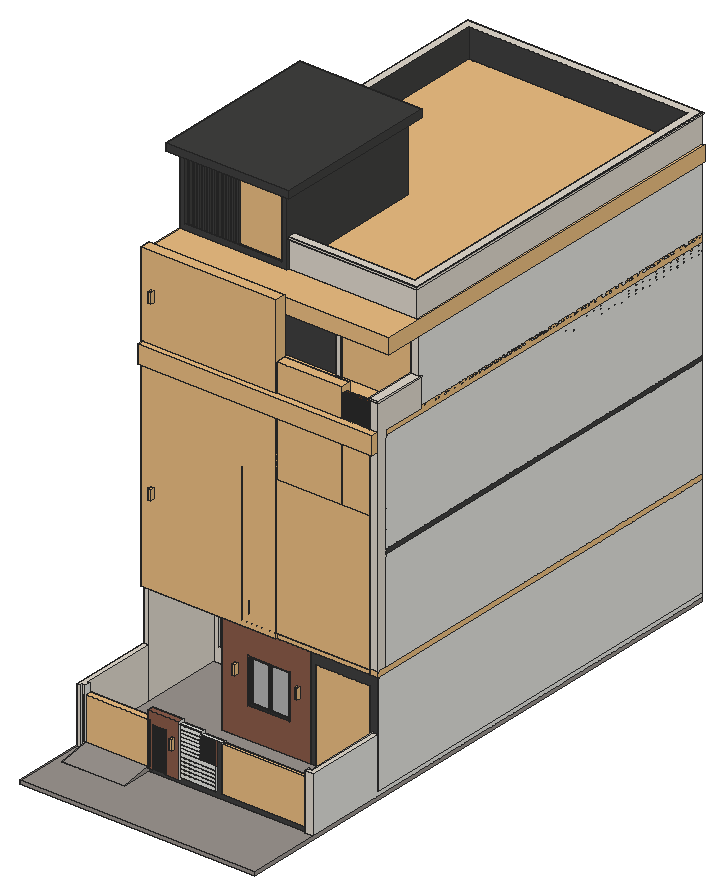
# SketchUp Ruby script. Lengths in inches.
U = 1.inch
M = Sketchup.active_model
def pt(a) = Geom::Point3d.new(a.map { |v| v * U })
def face(e, loops, mat)
  f = e.add_face(loops[0].map { |a| pt(a) })
  loops[1..].each { |l| e.add_face(l.map { |a| pt(a) }).erase! }
  f.material = f.back_material = mat if mat
  f
end
# faces: each face lists its corners as indices into pts; further lists are holes
def faces(e, pts, list, mat = nil) = list.each { |f| face(e, (f[0].is_a?(Array) ? f : [f]).map { |l| l.map { |i| pts[i] } }, mat) }
# xy, xz, yz: faces in a plane at the given z, y or x. An outline is a flat list of corners, or four numbers for a rectangle; further outlines are holes
def ring(l) = l.size == 4 ? [[l[0], l[1]], [l[2], l[1]], [l[2], l[3]], [l[0], l[3]]] : l.each_slice(2).to_a
def flat(e, list, mat, &to3) = list.each { |f| face(e, (f[0].is_a?(Array) ? f : [f]).map { |l| ring(l).map { |u, v| to3.(u, v) } }, mat) }
def xy(e, z, list, mat = nil) = flat(e, list, mat) { |x, y| [x, y, z] }
def xz(e, y, list, mat = nil) = flat(e, list, mat) { |x, z| [x, y, z] }
def yz(e, x, list, mat = nil) = flat(e, list, mat) { |y, z| [x, y, z] }
def lines(e, pts, list) = list.each { |a, b| e.add_line(pt(pts[a]), pt(pts[b])) }
# prism: a flat outline (further loops are holes) pulled along v
def prism(e, loops, v, mat = nil)
  f = face(e, loops, mat); d = Geom::Vector3d.new(v.map { |x| x * U })
  f.pushpull(f.normal.samedirection?(d) ? d.length : -d.length)
end
def box(e, o, s, mat = nil) = prism(e, [[o, [o[0] + s[0], o[1], o[2]], [o[0] + s[0], o[1] + s[1], o[2]], [o[0], o[1] + s[1], o[2]]]], [0, 0, s[2]], mat)
def at(x, y, z, deg = 0) = Geom::Transformation.translation(pt([x, y, z])) * Geom::Transformation.rotation(ORIGIN, Z_AXIS, deg.degrees)
def axes(o, x, y, z) = Geom::Transformation.new([*x, 0, *y, 0, *z, 0, *pt(o).to_a, 1])
def part(name) = M.definitions.add(name)
# library, detail: a bought-in or finely detailed component or shape, given as its bounding box
def library(name, o, s) = part(name).tap { |d| box(d.entities, o, s) }
def detail(e, o, s) = box(e.add_group.entities, o, s)
def put(e, d, t, mat = nil) = e.add_instance(d, t).tap { |i| i.material = mat if mat }
def group(e, t, mat = nil) = e.add_group.tap { |g| g.transformation = t; g.material = mat if mat }.entities
root = M.entities
M.materials.add("1448 AP 8253 RAVEN SONG").color = [64, 64, 63]
M.materials.add("Wall Light").color = [250, 218, 132]
M.materials.add("[0135_DarkGray]").color = [81, 81, 81]
M.materials.add("[Chris_Hair]").color = [71, 76, 74]
M.materials.add("[Concrete Stamped Ashlar]").color = [106, 67, 30]
M.materials.add("[Granite Tile]").color = [155, 148, 143]
M.materials.add("[Metal Seamed]").color = [61, 62, 60]
M.materials.add("[Steel Brushed Stainless]").color = [51, 51, 51]
M.materials.add("[Stone Vein Gray]").color = [63, 63, 63]
M.materials.add("[Tile Various Tan]").color = [223, 216, 204]
M.materials.add("[Translucent Glass Blue]1").color = [168, 168, 168]
M.materials.add("[Translucent Glass Gray]").color = [181, 181, 181]
M.materials.add("[Translucent Glass Gray]1").color = [128, 128, 128]
M.materials.add("[Wax 02]").color = [139, 92, 74]
M.materials.add("[Wood Veneer 01]").color = [91, 58, 35]
M.materials.add("[Wood Veneer 01]1").color = [120, 70, 37]
c1 = library("PF4VTX2R\#1",[0,-0.39,0],[145.67,4.18,85.83])
c2 = part("Group\#81")
prism(c2.entities,[[[8,8,0],[8,0,0],[0,0,0],[0,8,0]],[[4.25,3.75,0],[4.25,0.5,0],[7.5,0.5,0],[7.5,3.75,0]],[[0.5,7.5,0],[0.5,4.25,0],[3.75,4.25,0],[3.75,7.5,0]],[[5.625,4.25,0],[5.625,7.5,0],[4.25,7.5,0],[4.25,4.25,0]],[[7.5,7.5,0],[6.125,7.5,0],[6.125,4.25,0],[7.5,4.25,0]],[[0.5,3.75,0],[0.5,2.375,0],[3.75,2.375,0],[3.75,3.75,0]],[[0.5,0.5,0],[3.75,0.5,0],[3.75,1.875,0],[0.5,1.875,0]]],[0,0,3])
c3 = part("contemporary square jaali - swamy and co")
g1 = group(c3.entities,at(69.36,8.01,-1.33))
put(g1,c2,axes([24,1.28,40],[1,0,0],[0,0,1],[0,-0.42667,0]),"[Concrete Stamped Ashlar]")
put(g1,c2,axes([0,1.28,48],[1,0,0],[0,0,1],[0,-0.42667,0]),"[Concrete Stamped Ashlar]")
put(g1,c2,axes([8,1.28,40],[1,0,0],[0,0,1],[0,-0.42667,0]),"[Concrete Stamped Ashlar]")
put(g1,c2,axes([16,1.28,40],[1,0,0],[0,0,1],[0,-0.42667,0]),"[Concrete Stamped Ashlar]")
put(g1,c2,axes([8,1.28,48],[1,0,0],[0,0,1],[0,-0.42667,0]),"[Concrete Stamped Ashlar]")
put(g1,c2,axes([24,1.28,48],[1,0,0],[0,0,1],[0,-0.42667,0]),"[Concrete Stamped Ashlar]")
put(g1,c2,axes([16,1.28,48],[1,0,0],[0,0,1],[0,-0.42667,0]),"[Concrete Stamped Ashlar]")
put(g1,c2,axes([0,1.28,32],[1,0,0],[0,0,1],[0,-0.42667,0]),"[Concrete Stamped Ashlar]")
put(g1,c2,axes([8,1.28,24],[1,0,0],[0,0,1],[0,-0.42667,0]),"[Concrete Stamped Ashlar]")
put(g1,c2,axes([16,1.28,24],[1,0,0],[0,0,1],[0,-0.42667,0]),"[Concrete Stamped Ashlar]")
put(g1,c2,axes([24,1.28,24],[1,0,0],[0,0,1],[0,-0.42667,0]),"[Concrete Stamped Ashlar]")
put(g1,c2,axes([24,1.28,56],[1,0,0],[0,0,1],[0,-0.42667,0]),"[Concrete Stamped Ashlar]")
put(g1,c2,axes([16,1.28,8],[1,0,0],[0,0,1],[0,-0.42667,0]),"[Concrete Stamped Ashlar]")
put(g1,c2,axes([0,1.28,24],[1,0,0],[0,0,1],[0,-0.42667,0]),"[Concrete Stamped Ashlar]")
put(g1,c2,axes([0,1.28,16],[1,0,0],[0,0,1],[0,-0.42667,0]),"[Concrete Stamped Ashlar]")
put(g1,c2,axes([24,1.28,8],[1,0,0],[0,0,1],[0,-0.42667,0]),"[Concrete Stamped Ashlar]")
put(g1,c2,axes([8,1.28,16],[1,0,0],[0,0,1],[0,-0.42667,0]),"[Concrete Stamped Ashlar]")
put(g1,c2,axes([16,1.28,16],[1,0,0],[0,0,1],[0,-0.42667,0]),"[Concrete Stamped Ashlar]")
put(g1,c2,axes([24,1.28,16],[1,0,0],[0,0,1],[0,-0.42667,0]),"[Concrete Stamped Ashlar]")
put(g1,c2,axes([0,1.28,56],[1,0,0],[0,0,1],[0,-0.42667,0]),"[Concrete Stamped Ashlar]")
put(g1,c2,axes([24,1.28,32],[1,0,0],[0,0,1],[0,-0.42667,0]),"[Concrete Stamped Ashlar]")
put(g1,c2,axes([16,1.28,32],[1,0,0],[0,0,1],[0,-0.42667,0]),"[Concrete Stamped Ashlar]")
put(g1,c2,axes([0,1.28,40],[1,0,0],[0,0,1],[0,-0.42667,0]),"[Concrete Stamped Ashlar]")
put(g1,c2,axes([8,1.28,32],[1,0,0],[0,0,1],[0,-0.42667,0]),"[Concrete Stamped Ashlar]")
put(g1,c2,axes([0,1.28,0],[1,0,0],[0,0,1],[0,-0.42667,0]),"[Concrete Stamped Ashlar]")
put(g1,c2,axes([0,1.28,8],[1,0,0],[0,0,1],[0,-0.42667,0]),"[Concrete Stamped Ashlar]")
put(g1,c2,axes([16,1.28,56],[1,0,0],[0,0,1],[0,-0.42667,0]),"[Concrete Stamped Ashlar]")
put(g1,c2,axes([8,1.28,0],[1,0,0],[0,0,1],[0,-0.42667,0]),"[Concrete Stamped Ashlar]")
put(g1,c2,axes([16,1.28,0],[1,0,0],[0,0,1],[0,-0.42667,0]),"[Concrete Stamped Ashlar]")
put(g1,c2,axes([24,1.28,0],[1,0,0],[0,0,1],[0,-0.42667,0]),"[Concrete Stamped Ashlar]")
put(g1,c2,axes([8,1.28,56],[1,0,0],[0,0,1],[0,-0.42667,0]),"[Concrete Stamped Ashlar]")
put(g1,c2,axes([8,1.28,8],[1,0,0],[0,0,1],[0,-0.42667,0]),"[Concrete Stamped Ashlar]")
g2 = group(c3.entities,at(67.86,7.61,-2.83),"[Wood Veneer 01]")
xy(g2,0.5,[[0.5,0,34.5,2]])
xy(g2,1.5,[[1.5,0,33.5,2]])
xy(g2,65.5,[[1.5,0,33.5,2]])
xy(g2,66.5,[[0.5,0,34.5,2]])
xz(g2,0,[[[0.5,0.5,34.5,66.5],[1.5,1.5,33.5,65.5]]])
yz(g2,0.5,[[0,0.5,2,66.5]])
yz(g2,1.5,[[0,1.5,2,65.5]])
yz(g2,33.5,[[0,1.5,2,65.5]])
yz(g2,34.5,[[0,0.5,2,66.5]])
c4 = part("PENTEK_RP Fineline 50S_Sliding_DoorCase_E1")
box(c4.entities,[0,0,0],[1.51,3.66,99.27],"[0135_DarkGray]")
c5 = part("PENTEK_RP Fineline 50S_SlidingDooe_Case_E2")
box(c5.entities,[0,0,0],[96.25,3.66,1.51],"[0135_DarkGray]")
c6 = part("pentek_RP Fineline 50S_SlidingDoor_Case")
put(c6.entities,c4,at(97.76,0,0))
put(c6.entities,c5,at(1.51,0,0))
put(c6.entities,c4,at(0,0,0))
put(c6.entities,c5,at(1.51,0,97.76))
c7 = part("PENTEK_RP Fineline 50S_SlidingDoor_GlazingBead_2")
box(c7.entities,[0,0,0],[0.56,0.59,94.39],"[0135_DarkGray]")
c8 = part("PENTEK_RP Fineline 50S_SlidingDoor_Glass")
box(c8.entities,[0,0,0],[46.58,0.16,94.39],"[Translucent Glass Gray]1")
c9 = part("PENTEK_RP Fineline 50S_SlidingDoor_GlazingBead")
box(c9.entities,[0,0,0],[45.47,0.59,0.56],"[0135_DarkGray]")
c10 = part("PENTEK_RP Fineline 50S_SlidingDoor_Leaf_E1")
xy(c10.entities,0,[[0,0,0.93,1.97],[0.93,1.57,1.49,1.97]],"[0135_DarkGray]")
xy(c10.entities,96.25,[[0,0,0.93,0,0.93,1.57,1.49,1.57,1.49,1.97,0,1.97]],"[0135_DarkGray]")
xz(c10.entities,0,[[0,0,0.93,96.25]],"[0135_DarkGray]")
xz(c10.entities,1.57,[[0.93,0,1.49,95.32],[0.93,95.32,1.49,96.25]],"[0135_DarkGray]")
xz(c10.entities,1.97,[[0,0,1.49,96.25]],"[0135_DarkGray]")
yz(c10.entities,0,[[0,0,1.97,96.25]],"[0135_DarkGray]")
yz(c10.entities,0.93,[[0,0,1.57,0.93],[0,0.93,1.57,95.32],[0,95.32,1.57,96.25]],"[0135_DarkGray]")
yz(c10.entities,1.49,[[1.57,0,1.97,95.32],[1.57,95.32,1.97,96.25]],"[0135_DarkGray]")
c11 = part("PENTEK_RP Fineline 50S_SlidingDoor_Leaf_E2")
xy(c11.entities,0,[[0,0,0,1.57,0.56,1.57,0.56,1.97,46.02,1.97,46.02,1.57,46.58,1.57,46.58,0]],"[0135_DarkGray]")
xy(c11.entities,0.93,[[0,0,46.58,1.57]],"[0135_DarkGray]")
xy(c11.entities,1.49,[[0.56,1.57,46.02,1.97]],"[0135_DarkGray]")
xz(c11.entities,0,[[0,0,46.58,0.93]],"[0135_DarkGray]")
xz(c11.entities,1.57,[[0,0,0.56,0.93],[46.02,0,46.58,0.93],[0.56,0.93,46.02,1.49]],"[0135_DarkGray]")
xz(c11.entities,1.97,[[0.56,0,46.02,1.49]],"[0135_DarkGray]")
yz(c11.entities,0,[[0,0,1.57,0.93]],"[0135_DarkGray]")
yz(c11.entities,0.56,[[1.57,0,1.97,0.93],[1.57,0.93,1.97,1.49]],"[0135_DarkGray]")
yz(c11.entities,46.02,[[1.57,0,1.97,0.93],[1.57,0.93,1.97,1.49]],"[0135_DarkGray]")
yz(c11.entities,46.58,[[0,0,1.57,0.93]],"[0135_DarkGray]")
c12 = part("PENTEK_RP Fineline S_SlidingDoor_Leaf1")
put(c12.entities,c7,at(0.93,0,0.93))
put(c12.entities,c7,at(46.96,0,0.93))
put(c12.entities,c8,at(1.49,1.42,0.93))
put(c12.entities,c9,at(1.49,0,0.93))
put(c12.entities,c8,at(1.49,0.59,0.93))
put(c12.entities,c10,at(0,0,0))
put(c12.entities,c10,axes([48.44,0,0],[-1,0,0],[0,1,0],[0,0,1]))
put(c12.entities,c11,axes([0.93,0,96.25],[1,0,0],[0,1,0],[0,0,-1]))
put(c12.entities,c11,at(0.93,0,0))
put(c12.entities,c9,at(1.49,0,94.77))
c13 = part("PENTEK_RP Fineline 50S_SlidingDoor_Leaf2")
put(c13.entities,c8,at(1.49,1.42,0.93))
put(c13.entities,c9,at(1.49,0,94.77))
put(c13.entities,c7,at(46.96,0,0.93))
put(c13.entities,c8,at(1.49,0.59,0.93))
put(c13.entities,c7,at(0.93,0,0.93))
put(c13.entities,c10,at(0,0,0))
put(c13.entities,c10,axes([48.44,0,0],[-1,0,0],[0,1,0],[0,0,1]))
put(c13.entities,c9,at(1.49,0,0.93))
put(c13.entities,c11,axes([0.93,0,96.25],[1,0,0],[0,1,0],[0,0,-1]))
put(c13.entities,c11,at(0.93,0,0))
c14 = part("PENTEK_RP+Fineline+50S_Sliding_Door (1)")
put(c14.entities,c6,at(0,-1.88,-0.09))
put(c14.entities,c12,at(1.51,-2.27,1.42))
put(c14.entities,c13,at(49.32,-0.3,1.42))
c15 = library("AS-120-mm",[0,0,0],[49.44,4.72,66.14])
c16 = library("AS-120-mm\#1",[0,0,0],[49.44,4.72,60])
c17 = part("หน้าต่าง3บาน")
xy(c17.entities,42.78,[[77.6875,12.74,148.55,16.68]])
xy(c17.entities,43.96,[[78.87,12.74,147.37,12.74,147.37,14.71,125.72,14.71,125.72,13.13,100.52,13.13,100.52,14.71,78.87,14.71],[100.52,13.13,102.88,14.71],[123.36,13.13,125.72,14.71],[102.49,14.71,123.75,14.71,123.75,16.28,147.37,16.28,147.37,16.68,78.87,16.68,78.87,16.28,102.49,16.28]])
xy(c17.entities,45.93,[[102.49,13.13,123.75,13.92],[102.49,13.92,123.75,14.71],[80.84,14.71,100.52,15.49],[125.72,14.71,145.4,15.49],[80.84,15.49,100.52,16.28],
  [125.72,15.49,145.4,16.28]])
xy(c17.entities,83.09,[[102.49,13.13,123.75,13.92],[102.49,13.92,123.75,14.71],[80.84,14.71,100.52,15.49],[125.72,14.71,145.4,15.49],[80.84,15.49,100.52,16.28],
  [125.72,15.49,145.4,16.28]])
xy(c17.entities,84.91,[[78.87,12.74,78.87,14.71,100.52,14.71,100.52,13.13,125.72,13.13,125.72,14.71,147.37,14.71,147.37,12.74],[100.52,13.13,125.72,14.71],[102.49,14.71,102.49,16.28,78.87,16.28,78.87,16.68,147.37,16.68,147.37,16.28,123.75,16.28,123.75,14.71],[78.87,14.71,102.49,16.28]])
xy(c17.entities,86.09,[[77.6875,12.74,148.55,16.68]])
xz(c17.entities,12.74,[[[77.6875,42.78,148.55,86.09],[78.87,43.96,147.37,84.91]]])
xz(c17.entities,13.13,[[[100.52,43.96,125.72,84.91],[102.49,45.93,123.75,83.09]]])
xz(c17.entities,13.92,[[102.49,45.93,123.75,83.09]],"[Translucent Glass Blue]1")
xz(c17.entities,14.71,[[78.87,43.96,100.52,43.96,100.52,45.93,80.84,45.93,80.84,83.09,100.52,83.09,100.52,84.91,78.87,84.91],[100.52,43.96,102.49,84.91],[102.49,43.96,123.75,45.93],[125.72,43.96,147.37,43.96,147.37,84.91,125.72,84.91,125.72,83.09,145.4,83.09,145.4,45.93,125.72,45.93],[102.49,83.09,123.75,84.91]])
xz(c17.entities,15.49,[[80.44,82.9375,80.84,83.73]])
xz(c17.entities,15.49,[[80.84,45.93,100.52,83.09],[125.72,45.93,145.4,83.09]],"[Translucent Glass Blue]1")
xz(c17.entities,16.28,[[[78.87,43.96,102.49,84.91],[80.84,45.93,100.52,83.09]],[[123.75,43.96,147.37,84.91],[125.72,45.93,145.4,83.09]]])
xz(c17.entities,16.68,[[[77.6875,42.78,148.55,86.09],[78.87,43.96,147.37,84.91]]])
yz(c17.entities,77.6875,[[12.74,42.78,16.68,86.09]])
yz(c17.entities,78.87,[[12.74,43.96,14.71,84.91],[16.28,43.96,16.68,84.91]])
yz(c17.entities,80.84,[[14.71,45.93,15.49,83.09],[15.49,45.93,16.28,83.09]])
yz(c17.entities,100.52,[[13.13,43.96,14.71,84.91],[14.71,45.93,15.49,83.09],[15.49,45.93,16.28,83.09]])
yz(c17.entities,102.49,[[14.71,43.96,16.28,84.91],[13.13,45.93,13.92,83.09],[13.92,45.93,14.71,83.09]])
yz(c17.entities,123.75,[[14.71,43.96,16.28,84.91],[13.13,45.93,13.92,83.09],[13.92,45.93,14.71,83.09]])
yz(c17.entities,125.72,[[13.13,43.96,14.71,84.91],[14.71,45.93,15.49,83.09],[15.49,45.93,16.28,83.09]])
yz(c17.entities,145.4,[[14.71,45.93,15.49,83.09],[15.49,45.93,16.28,83.09]])
yz(c17.entities,147.37,[[12.74,43.96,14.71,84.91],[16.28,43.96,16.68,84.91]])
yz(c17.entities,148.55,[[12.74,42.78,16.68,86.09]])
# 1 loose lines left out
c18 = library("Curtains",[0,0,0],[121.73,8.19,117.22])
c19 = library("Component",[1.03,-1.63,0],[72.41,6.81,50.39])
c20 = library("11",[-5.64,-5.64,-13.23],[15.28,15.28,13.23])
c21 = library("WALL LIGHT 69",[4.19,4.05,-8.78],[4.61,5.7,17.13])
c22 = library("porte moderne noir",[57.21,0.32,0],[43.81,4.72,87.03])
c23 = part("Group\#3")
g3 = group(c23.entities,at(0,3,0))
prism(g3,[[[9,0,0],[0,0,0],[0,0,72],[9,0,72]],[[0.75,0,71.25],[0.75,0,0.75],[8.25,0,0.75],[8.25,0,71.25]]],[0,-1,0])
g4 = group(g3,at(0.75,-0.26,0.75),"[Translucent Glass Gray]")
box(g4,[0,-0.47,0],[7.5,0.47,70.5])
c24 = part("Group\#8")
g5 = group(c24.entities,at(0,1.75,0))
prism(g5,[[[21,0,0],[0,0,0],[0,0,50],[21,0,50]],[[20,0,49],[1,0,49],[1,0,1],[20,0,1]]],[0,-1.5,0])
g6 = group(g5,at(1,-0.5,1),"[Translucent Glass Gray]")
box(g6,[0,-0.47,0],[19,0.47,48])
c25 = library("Group\#93",[0,-4.51,0],[63,7.09,108])
c26 = library("Group\#12",[0,0,0],[270,480,6])
c27 = library("Jaali+Partition",[0,0,0],[29.75,4.875,91.45])
c28 = library("Group\#15",[-15,-12.5,0],[147,12.5,163])
c29 = library("Group\#17",[0,0,0],[75,12,279])
c30 = library("Group\#18",[0,-3.5,0],[74,3.5,102])
c31 = library("Group\#20",[-2.91,0,-6],[155.91,13,360])
c32 = part("1")
prism(c32.entities,[[[2,-1,0],[2,1,0],[2,1,48],[2,4,48],[2,4,50],[2,-1,50]]],[-2,0,0])
c33 = library("Group\#72",[0,-2,0],[89,2,34])
c34 = part("Group\#80")
box(c34.entities,[0,-0.5,0],[24,0.5,32.25])
c35 = library("Group\#22",[0,-12.5,0],[72,12.5,15.01])
c36 = library("Group\#59",[0,-81,-11.98],[270,489,20.98])
c37 = library("Group\#92",[0,0,0],[75.39,1.25,93])
c38 = library("Group\#62",[0,-51,-11.98],[273,468,17.98])
c39 = part("2")
box(c39.entities,[0,0,0],[3,2,70])
c40 = part("8")
box(c40.entities,[0,0.25,0],[0.5,0.25,24.5])
c41 = part("9")
box(c41.entities,[0,0,0],[0.25,0.25,48.1875])
c42 = library("Group\#151",[0,0,0],[124.17,4.81,62])
g7 = group(root,at(9.27,183,0))
put(g7,c1,axes([6.18,58,483],[0.78486,0,0],[0,1,0],[0,0,0.8156]))
put(g7,c3,axes([-112.47,4.39,256.23],[1.73559,0,0],[0,1,0],[0,0,1.81818]))
put(g7,c14,axes([27.81,76.22,252.09],[0.90267,0,0],[0,1,0],[0,0,0.96704]))
put(g7,c14,axes([35.72,70.22,376.61],[0.63625,0,0],[0,1,0],[0,0,0.80042]))
put(g7,c15,at(197.76,74,282))
put(g7,c16,at(176.13,14,156),"[Metal Seamed]")
put(g7,c17,axes([-31.86,-4.51,96.73],[1.04648,0,0],[0,1.35,0],[0,0,1.38545]),"[Metal Seamed]")
put(g7,c18,axes([22.45,72,378.94],[0.721,0,0],[0,0.7,0],[0,0,0.7]))
put(g7,c18,axes([19.71,81,252],[0.85655,0,0],[0,0.7,0],[0,0,0.861]))
put(g7,c18,axes([177.7,81,273.25],[0.721,0,0],[0,0.7,0],[0,0,0.7]))
put(g7,c18,axes([43.39,21,140.04],[0.721,0,0],[0,0.7,0],[0,0,0.7]))
put(g7,c18,axes([157.61,21,139.96],[0.721,0,0],[0,0.7,0],[0,0,0.7]))
put(g7,c18,axes([110.14,9,21.49],[0.62727,0,0],[0,0.609,0],[0,0,0.609]))
put(g7,c18,axes([192.39,9,0],[0.62727,0,0],[0,0.7,0],[0,0,0.973]))
put(g7,c18,axes([9.27,105,0],[0.721,0,0],[0,0.7,0],[0,0,0.812]))
put(g7,c19,axes([5.23,-95,0],[1.0816,0,0],[0,1,0],[0,0,1]))
put(g7,c20,at(28.18,22,121.38))
put(g7,c20,at(66.7,22,121.38))
put(g7,c21,axes([107.17,-103.32,34.52],[0.7,0,0],[0,0.7,0],[0,0,0.7]))
put(g7,c21,axes([6.26,-7.82,223.42],[0.7,0,0],[0,0.7,0],[0,0,0.7]))
put(g7,c21,axes([6.26,-7.82,432.14],[0.7,0,0],[0,0.7,0],[0,0,0.7]))
put(g7,c21,axes([137.82,65.18,317.875],[0.7,0,0],[0,0.7,0],[0,0,0.7]))
put(g7,c21,axes([234.6,1.68,184.42],[0.7,0,0],[0,0.7,0],[0,0,0.7]))
put(g7,c21,axes([179.03,-6.82,71.52],[0.7,0,0],[0,0.7,0],[0,0,0.7]))
put(g7,c21,axes([105.28,-6.82,71.52],[0.7,0,0],[0,0.7,0],[0,0,0.7]))
g8 = group(g7,at(0,0,0))
xy(g8,0,[[0,0,0,480,278.1,480,278.1,1,268.83,1,268.83,471,9.27,471,9.27,105,27.81,105,27.81,96,6.18,96,6.18,0],[92.7,0,92.7,96,71.07,96,71.07,105,101.97,105,101.97,9,203.94,9,203.94,1,197.76,1,197.76,0]])
xy(g8,18,[[12.36,96,21.63,105],[77.25,96,86.52,105]])
xy(g8,36,[[123.6,0,173.04,9]],"[Wax 02]")
xy(g8,90,[[12.36,96,21.63,105],[27.81,96,71.07,105],[77.25,96,86.52,105]])
xy(g8,90,[[123.6,0,173.04,9]],"[Wax 02]")
xy(g8,108,[[203.94,1,268.83,9]])
xy(g8,120,[[[0,0,6.18,0,6.18,96,92.7,96,92.7,0,197.76,0,197.76,1,278.1,1,278.1,480,0,480],[101.97,9,101.97,105,9.27,105,9.27,471,268.83,471,268.83,9]]])
xz(g8,0,[[0,0,6.18,120]],"[Tile Various Tan]")
xz(g8,0,[[[92.7,0,197.76,120],[123.6,36,173.04,90]]],"[Wax 02]")
xz(g8,1,[[197.76,0,203.94,0,203.94,108,268.83,108,268.83,0,278.1,0,278.1,120,197.76,120]])
xz(g8,9,[[[101.97,0,101.97,120,268.83,120,268.83,108,203.94,108,203.94,0],[123.6,36,173.04,90]]])
xz(g8,96,[[[6.18,0,27.81,0,27.81,90,71.07,90,71.07,0,92.7,0,92.7,120,6.18,120],[77.25,18,86.52,90],[12.36,18,21.63,90]]],"[Tile Various Tan]")
xz(g8,105,[[[9.27,0,9.27,120,101.97,120,101.97,0,71.07,0,71.07,90,27.81,90,27.81,0],[77.25,18,86.52,90],[12.36,18,21.63,90]]])
xz(g8,471,[[9.27,0,268.83,120]])
xz(g8,480,[[0,0,278.1,120]])
yz(g8,0,[[0,0,480,120]])
yz(g8,6.18,[[0,0,96,120]],"[Tile Various Tan]")
yz(g8,9.27,[[105,0,471,120]])
yz(g8,12.36,[[96,18,105,90]])
yz(g8,21.63,[[96,18,105,90]])
yz(g8,27.81,[[96,0,105,90]])
yz(g8,71.07,[[96,0,105,90]])
yz(g8,77.25,[[96,18,105,90]])
yz(g8,86.52,[[96,18,105,90]])
yz(g8,92.7,[[0,0,96,120]],"[Wax 02]")
yz(g8,101.97,[[9,0,105,120]])
yz(g8,123.6,[[0,36,9,90]],"[Wax 02]")
yz(g8,173.04,[[0,36,9,90]],"[Wax 02]")
yz(g8,197.76,[[0,0,1,120]])
yz(g8,203.94,[[1,0,9,108]])
yz(g8,268.83,[[1,0,9,108],[9,0,471,120]])
yz(g8,278.1,[[1,0,480,120]])
put(g8,c22,axes([-28.67,97.68,0],[0.98737,0,0],[0,1,0],[0,0,1.03407]))
put(g8,c23,axes([12.36,96,18],[1.03,0,0],[0,1,0],[0,0,1]),"[Wood Veneer 01]")
put(g8,c23,axes([77.25,96,18],[1.03,0,0],[0,1,0],[0,0,1]),"[Wood Veneer 01]")
g9 = group(g8,at(123.6,4,36),"[Steel Brushed Stainless]")
g10 = group(g9,at(0,0,0))
prism(g10,[[[49.44,0,0],[0,0,0],[0,0,54],[49.44,0,54]],[[23.69,0,2],[23.69,0,52],[2.06,0,52],[2.06,0,2]],[[25.75,0,2],[47.38,0,2],[47.38,0,52],[25.75,0,52]]],[0,-2,0])
put(g10,c24,axes([2.06,-2,2],[1.03,0,0],[0,1,0],[0,0,1]))
put(g10,c24,axes([25.75,-2,2],[1.03,0,0],[0,1,0],[0,0,1]))
g11 = group(g8,at(197.76,1,0),"[Stone Vein Gray]")
prism(g11,[[[80.34,0,0],[71.07,0,0],[71.07,0,108],[6.18,0,108],[6.18,0,0],[0,0,0],[0,0,120],[80.34,0,120]]],[0,-1,0])
put(g8,c25,axes([203.94,4.51,0],[1.03,0,0],[0,1,0],[0,0,1]),"[Steel Brushed Stainless]")
put(g7,c26,axes([0,0,120],[1.03,0,0],[0,1,0],[0,0,1]),"1448 AP 8253 RAVEN SONG")
g12 = group(g7,at(0,0,126))
xy(g12,0,[[[0,12,278.1,480],[9.27,21,268.83,471]]])
xy(g12,30,[[49.44,12,123.6,21],[176.13,12,225.57,21]])
xy(g12,90,[[49.44,12,123.6,21],[176.13,12,225.57,21]])
xy(g12,120,[[[0,12,278.1,480],[9.27,21,268.83,471]]])
xz(g12,12,[[[0,0,278.1,120],[49.44,30,123.6,90],[176.13,30,225.57,90]]],"[Tile Various Tan]")
xz(g12,21,[[[9.27,0,268.83,120],[49.44,30,123.6,90],[176.13,30,225.57,90]]])
xz(g12,471,[[9.27,0,268.83,120]])
xz(g12,480,[[0,0,278.1,120]])
yz(g12,0,[[12,0,480,120]])
yz(g12,9.27,[[21,0,471,120]])
yz(g12,49.44,[[12,30,21,90]])
yz(g12,123.6,[[12,30,21,90]])
yz(g12,176.13,[[12,30,21,90]])
yz(g12,225.57,[[12,30,21,90]])
yz(g12,268.83,[[21,0,471,120]])
yz(g12,278.1,[[12,0,480,120]])
g13 = group(g12,at(0,12,0),"[Tile Various Tan]")
xy(g13,-6,[[268.83,-12,278.1,0]])
xy(g13,252,[[268.83,0,278.1,51]])
xy(g13,286.5,[[267.8,-13,267.8,51,268.83,51,268.83,-12,278.1,-12,278.1,51,279.13,51,279.13,-13]])
xy(g13,288,[[267.8,-13,279.13,51]])
xz(g13,-13,[[267.8,286.5,279.13,288]])
xz(g13,-12,[[268.83,-6,278.1,286.5]],"[Tile Various Tan]")
xz(g13,0,[[268.83,-6,278.1,252]])
xz(g13,51,[[268.83,252,278.1,288],[267.8,286.5,268.83,288],[278.1,286.5,279.13,288]])
yz(g13,267.8,[[-13,286.5,51,288]])
yz(g13,268.83,[[-12,-6,-12,286.5,51,286.5,51,252,0,252,0,-6]],"[Tile Various Tan]")
yz(g13,278.1,[[-12,-6,0,-6,0,252,51,252,51,286.5,-12,286.5]])
yz(g13,279.13,[[-13,286.5,51,288]])
# 5 loose lines left out
put(g13,c27,axes([234.84,-12,126],[1.14262,0,0],[0,1,0],[0,0,1.15906]))
put(g13,c28,axes([132.87,0,0],[1.03,0,0],[0,1,0],[0,0,1]),"[Stone Vein Gray]")
put(g13,c29,axes([157.59,-12,9],[1.03,0,0],[0,1,0],[0,0,1]))
put(g13,c30,axes([176.13,0,9],[1.03,0,0],[0,1,0],[0,0,1]),"[Wood Veneer 01]1")
g14 = group(g13,at(176.13,0,9),"[Tile Various Tan]")
detail(g14,[0,-10.5,0],[92.7,10.5,117])
put(g13,c31,axes([0,-13,0],[1.03,0,0],[0,1,0],[0,0,1]))
g15 = group(g13,at(132.87,-13,0),"[Tile Various Tan]")
box(g15,[-108.15,1,0],[108.15,11,8.99])
g16 = group(g13,at(234.84,-12,232),"[Wood Veneer 01]1")
xy(g16,0,[[0,3,33.99,6]])
xy(g16,48,[[0,3,33.99,6]])
xz(g16,3,[[0,0,33.99,48]])
xz(g16,6,[[0,0,33.99,48]])
yz(g16,0,[[3,0,6,48]])
yz(g16,33.99,[[3,0,6,48]])
put(g16,c32,axes([0,2,0],[1.11023,0,0],[0,1,0],[0,0,1]))
put(g16,c32,axes([2.65,2,0],[1.11023,0,0],[0,1,0],[0,0,1]))
put(g16,c32,axes([5.29,2,0],[1.11023,0,0],[0,1,0],[0,0,1]))
put(g16,c32,axes([7.94,2,0],[1.11023,0,0],[0,1,0],[0,0,1]))
put(g16,c32,axes([10.59,2,0],[1.11023,0,0],[0,1,0],[0,0,1]))
put(g16,c32,axes([13.24,2,0],[1.11023,0,0],[0,1,0],[0,0,1]))
put(g16,c32,axes([15.88,2,0],[1.11023,0,0],[0,1,0],[0,0,1]))
put(g16,c32,axes([18.53,2,0],[1.11023,0,0],[0,1,0],[0,0,1]))
put(g16,c32,axes([21.18,2,0],[1.11023,0,0],[0,1,0],[0,0,1]))
put(g16,c32,axes([23.83,2,0],[1.11023,0,0],[0,1,0],[0,0,1]))
put(g16,c32,axes([26.47,2,0],[1.11023,0,0],[0,1,0],[0,0,1]))
put(g16,c32,axes([29.12,2,0],[1.11023,0,0],[0,1,0],[0,0,1]))
put(g16,c32,axes([31.77,2,0],[1.11023,0,0],[0,1,0],[0,0,1]))
put(g13,c33,axes([25.75,-6,126],[1.03,0,0],[0,1,0],[0,0,1]))
g17 = group(g13,at(25.75,-9,252))
g18 = group(g17,at(0,0.5,32),"[Steel Brushed Stainless]")
prism(g18,[[[0,0,2],[0,0,0],[0,-0.75,0],[0,-0.75,0.25],[0,-1.25,0.25],[0,-1.25,0],[0,-2,0],[0,-2,2]]],[88.58,0,0])
g19 = group(g17,at(0,-0.25,0),"[Translucent Glass Gray]")
xy(g19,0,[[0,-0.47,88.58,0]])
xy(g19,32.25,[[0,-0.47,88.58,0]])
xz(g19,-0.47,[[0,0,88.58,32.25]])
xz(g19,0,[[0,0,88.58,32.25]])
yz(g19,0,[[-0.47,0,0,32.25]])
yz(g19,88.58,[[-0.47,0,0,32.25]])
g20 = group(g17,at(110.12,-2,0))
g21 = group(g20,at(0,2,32),"[Steel Brushed Stainless]")
prism(g21,[[[0,0,2],[0,0,0],[0,-0.75,0],[0,-0.75,0.25],[0,-1.25,0.25],[0,-1.25,0],[0,-2,0],[0,-2,2]]],[21.72,0,0])
put(g20,c34,axes([0,1.25,0],[0.905,0,0],[0,1,0],[0,0,1]),"[Translucent Glass Gray]")
put(g13,c34,axes([177.6875,-7.55,126],[1.93069,0,0],[0,1,0],[0,0,1]),"[Translucent Glass Gray]")
g22 = group(g13,at(177.6875,-6.8,158),"[Steel Brushed Stainless]")
prism(g22,[[[0,0,2],[0,0,0],[0,-0.75,0],[0,-0.75,0.25],[0,-1.25,0.25],[0,-1.25,0],[0,-2,0],[0,-2,2]]],[46.34,0,0])
put(g12,c35,axes([48.7,12,8.99],[1.06111,0,0],[0,1,0],[0,0,1.02]),"[Wood Veneer 01]1")
g23 = group(g7,at(0,12,246),"1448 AP 8253 RAVEN SONG")
box(g23,[0,0,0],[278.1,468,6])
g24 = group(g7,at(0,12,252))
xy(g24,0,[[0,0,0,468,278.1,468,278.1,0,271.92,0,271.92,60,117.42,60,117.42,69,268.83,69,268.83,459,9.27,459,9.27,69,27.81,69,27.81,60,6.18,60,6.18,0]])
xy(g24,30,[[197.76,60,247.2,69]])
xy(g24,96,[[27.81,60,117.42,69],[197.76,60,247.2,69]])
xy(g24,120,[[[0,0,6.18,0,6.18,60,271.92,60,271.92,0,278.1,0,278.1,468,0,468],[9.27,69,268.83,459]]])
xz(g24,0,[[0,0,6.18,120],[271.92,0,278.1,120]])
xz(g24,60,[[[6.18,0,27.81,0,27.81,96,117.42,96,117.42,0,271.92,0,271.92,120,6.18,120],[197.76,30,247.2,96]]],"[Tile Various Tan]")
xz(g24,69,[[[9.27,0,9.27,120,268.83,120,268.83,0,117.42,0,117.42,96,27.81,96,27.81,0],[197.76,30,247.2,96]]])
xz(g24,459,[[9.27,0,268.83,120]])
xz(g24,468,[[0,0,278.1,120]])
yz(g24,0,[[0,0,468,120]])
yz(g24,6.18,[[0,0,60,120]])
yz(g24,9.27,[[69,0,459,120]])
yz(g24,27.81,[[60,0,69,96]])
yz(g24,117.42,[[60,0,69,96]])
yz(g24,197.76,[[60,30,69,96]])
yz(g24,247.2,[[60,30,69,96]])
yz(g24,268.83,[[69,0,459,120]])
yz(g24,271.92,[[0,0,60,120]])
yz(g24,278.1,[[0,0,468,120]])
put(g7,c36,axes([0,72,372],[1.03,0,0],[0,1,0],[0,0,1]),"1448 AP 8253 RAVEN SONG")
g25 = group(g7,at(0,12,378))
xy(g25,0,[[0,0,0,468,278.1,468,278.1,51,185.4,51,185.4,49,179.22,49,179.22,50,117.42,50,117.42,51,98.88,51,98.88,60,268.83,60,268.83,459,9.27,459,9.27,60,37.08,60,37.08,51,6.18,51,6.18,0]])
xy(g25,36,[[267.8,49,278.1,51]])
xy(g25,78,[[37.08,51,98.88,60]])
xy(g25,93,[[[0,0,6.18,0,6.18,51,117.42,51,117.42,50,179.22,50,179.22,49,185.4,49,185.4,51,267.8,51,267.8,49,278.1,49,278.1,468,0,468],[9.27,60,268.83,459]]])
xz(g25,0,[[0,0,6.18,93]])
xz(g25,49,[[179.22,0,185.4,93],[267.8,36,278.1,93]],"[Tile Various Tan]")
xz(g25,50,[[117.42,0,179.22,93]],"[Stone Vein Gray]")
xz(g25,51,[[185.4,0,278.1,0,278.1,36,267.8,36,267.8,93,185.4,93]])
xz(g25,51,[[6.18,0,37.08,0,37.08,78,98.88,78,98.88,0,117.42,0,117.42,93,6.18,93]],"[Tile Various Tan]")
xz(g25,60,[[9.27,0,9.27,93,268.83,93,268.83,0,98.88,0,98.88,78,37.08,78,37.08,0]])
xz(g25,459,[[9.27,0,268.83,93]])
xz(g25,468,[[0,0,278.1,93]])
yz(g25,0,[[0,0,468,93]])
yz(g25,6.18,[[0,0,51,93]])
yz(g25,9.27,[[60,0,459,93]])
yz(g25,37.08,[[51,0,60,78]])
yz(g25,98.88,[[51,0,60,78]])
yz(g25,117.42,[[50,0,51,93]])
yz(g25,179.22,[[49,0,50,93]])
yz(g25,185.4,[[49,0,51,93]])
yz(g25,267.8,[[49,36,51,93]])
yz(g25,268.83,[[60,0,459,93]])
yz(g25,278.1,[[51,0,468,0,468,93,49,93,49,36,51,36]])
put(g25,c37,axes([185.4,49.5,0],[1.09303,0,0],[0,1,0],[0,0,1]))
put(g7,c38,axes([0,63,471],[1.03,0,0],[0,1,0],[0,0,1]),"1448 AP 8253 RAVEN SONG")
g26 = group(g7,at(0,57,477),"1448 AP 8253 RAVEN SONG")
xy(g26,0,[[[0,-3,0,423,278.1,423,278.1,0,126.69,0,126.69,-3],[126.69,9,268.83,9,268.83,414,9.27,414,9.27,177,126.69,177],[6.18,6,120.51,171]]])
xy(g26,6,[[6.18,-3,120.51,6]])
xy(g26,30.875,[[126.81,0,277.98,0.25]],"[Tile Various Tan]")
xy(g26,31.875,[[126.81,0,277.98,0.25]],"[Tile Various Tan]")
xy(g26,32,[[126.69,-2,126.69,0,278.1,0,278.1,423,280.16,423,280.16,-2]],"[Tile Various Tan]")
xy(g26,34,[[126.69,-2,280.16,-2,280.16,423,278.1,423,278.1,0,126.69,0],[126.69,0,278.1,0,278.1,423,0,423,0,177,9.27,177,9.27,414,268.83,414,268.83,9,126.69,9]],"[Tile Various Tan]")
xy(g26,76,[[6.18,-3,120.51,6]])
xy(g26,82,[[[0,-3,126.69,177],[6.18,6,120.51,171]]])
xz(g26,-3,[[[0,0,126.69,82],[6.18,6,120.51,76]]])
xz(g26,-2,[[126.69,32,280.16,34]],"[Tile Various Tan]")
xz(g26,0,[[126.69,32,278.1,34]])
xz(g26,0,[[[126.69,0,278.1,32],[126.81,30.875,277.98,31.875]]],"[Tile Various Tan]")
xz(g26,0.25,[[126.81,30.875,277.98,31.875]],"[Tile Various Tan]")
xz(g26,6,[[6.18,0,120.51,6],[6.18,76,120.51,82]])
xz(g26,9,[[126.69,0,268.83,34]])
xz(g26,171,[[6.18,0,120.51,82]])
xz(g26,177,[[9.27,0,9.27,34,0,34,0,82,126.69,82,126.69,0]])
xz(g26,414,[[9.27,0,268.83,34]])
xz(g26,423,[[0,0,278.1,34],[278.1,32,280.16,34]])
yz(g26,0,[[-3,0,-3,82,177,82,177,34,423,34,423,0]])
yz(g26,6.18,[[6,0,171,0,171,82,6,82,6,76,-3,76,-3,6,6,6]])
yz(g26,9.27,[[177,0,414,34]])
yz(g26,120.51,[[6,0,171,82],[-3,6,6,76]])
yz(g26,126.69,[[-3,0,0,0,0,32,-2,32,-2,34,9,34,9,0,177,0,177,82,-3,82],[-2,32,0,34]])
yz(g26,126.81,[[0,30.875,0.25,31.875]],"[Tile Various Tan]")
yz(g26,268.83,[[9,0,414,34]])
yz(g26,277.98,[[0,30.875,0.25,31.875]],"[Tile Various Tan]")
yz(g26,278.1,[[0,32,423,34]])
yz(g26,278.1,[[0,0,423,32]],"[Tile Various Tan]")
yz(g26,280.16,[[-2,32,423,34]],"[Tile Various Tan]")
put(g26,c39,axes([7.72,-1.5,6],[1.03,0,0],[0,1,0],[0,0,1]))
put(g26,c39,axes([13.45,-1.5,6],[1.03,0,0],[0,1,0],[0,0,1]))
put(g26,c39,axes([19.17,-1.5,6],[1.03,0,0],[0,1,0],[0,0,1]))
put(g26,c39,axes([24.89,-1.5,6],[1.03,0,0],[0,1,0],[0,0,1]))
put(g26,c39,axes([30.62,-1.5,6],[1.03,0,0],[0,1,0],[0,0,1]))
put(g26,c39,axes([36.34,-1.5,6],[1.03,0,0],[0,1,0],[0,0,1]))
put(g26,c39,axes([42.0625,-1.5,6],[1.03,0,0],[0,1,0],[0,0,1]))
put(g26,c39,axes([47.79,-1.5,6],[1.03,0,0],[0,1,0],[0,0,1]))
put(g26,c39,axes([53.51,-1.5,6],[1.03,0,0],[0,1,0],[0,0,1]))
put(g26,c39,axes([59.23,-1.5,6],[1.03,0,0],[0,1,0],[0,0,1]))
put(g26,c39,axes([64.95,-1.5,6],[1.03,0,0],[0,1,0],[0,0,1]))
g27 = group(g26,at(0,-3,82))
box(g27,[-9.27,-9,0],[145.23,198,9])
g28 = group(g26,at(126.81,0,30.875),"Wall Light")
box(g28,[0,0,0],[151.16,0.25,1],"Wall Light")
g29 = group(g7,at(0,0,0))
xy(g29,-6,[[0,-99,0,480,278.1,480,278.1,-96,267.8,-96,267.8,-95,8.24,-95,8.24,-97,4.12,-97,4.12,-99]])
xy(g29,-2,[[82.4,-96.5,87.55,-95],[104.03,-96.5,119.48,-95],[87.55,-95,104.03,-95,104.03,-94,87.81,-94,87.81,-94.25,87.55,-94.25]])
xy(g29,0,[[8.24,-95,82.4,-95,82.4,-90,168.92,-90,168.92,-95,267.8,-95,267.8,-90,271.92,-90,271.92,0,278.1,0,278.1,480,0,480,0,0,6.18,0,6.18,-90,8.24,-90]],"[Granite Tile]")
xy(g29,1,[[119.48,-96,162.74,-95]])
xy(g29,6,[[119.48,-96,162.74,-95.75]])
xy(g29,6.25,[[119.48,-96,162.74,-95.75]])
xy(g29,10.25,[[119.48,-96,162.74,-95.75]])
xy(g29,10.5,[[119.48,-96,162.74,-95.75]])
xy(g29,14.5,[[119.48,-96,162.74,-95.75]])
xy(g29,14.75,[[119.48,-96,162.74,-95.75]])
xy(g29,18.75,[[119.48,-96,162.74,-95.75]])
xy(g29,19,[[119.48,-96,162.74,-95.75]])
xy(g29,23,[[119.48,-96,162.74,-95.75]])
xy(g29,23.25,[[119.48,-96,162.74,-95.75]])
xy(g29,27.75,[[119.48,-96,144.2,-95],[144.2,-96,162.74,-95]])
xy(g29,46,[[87.55,-96.5,104.03,-94]],"[Wax 02]")
xy(g29,54,[[144.2,-95,168.92,-90]])
xy(g29,57,[[119.48,-95,144.2,-90]])
xy(g29,60,[[0,-99,4.12,-99,4.12,-97,8.24,-97,8.24,-90,6.18,-90,6.18,0,0,0],[267.8,-96,278.1,-96,278.1,0,271.92,0,271.92,-90,267.8,-90]],"[Tile Various Tan]")
xy(g29,60,[[82.4,-96.5,119.48,-90]],"[Wax 02]")
xz(g29,-99,[[0,-6,4.12,60]],"[Tile Various Tan]")
xz(g29,-97,[[4.12,-6,8.24,60]],"[Tile Various Tan]")
xz(g29,-96.5,[[82.4,-2,87.55,-2,87.55,46,104.03,46,104.03,-2,119.48,-2,119.48,60,82.4,60]],"[Wax 02]")
xz(g29,-96,[[119.48,1,162.74,6],[119.48,6.25,162.74,10.25],[119.48,10.5,162.74,14.5],[119.48,14.75,162.74,18.75],[119.48,19,162.74,23],
  [119.48,23.25,162.74,27.75]])
xz(g29,-96,[[267.8,-6,278.1,60]],"[Tile Various Tan]")
xz(g29,-95.75,[[119.48,6,162.74,6.25],[119.48,10.25,162.74,10.5],[119.48,14.5,162.74,14.75],[119.48,18.75,162.74,19],[119.48,23,162.74,23.25]])
xz(g29,-95,[[119.48,28,144.2,57],[144.2,28,162.74,54]])
xz(g29,-95,[[82.4,-6,267.8,-6,267.8,0,168.92,0,168.92,54,162.74,54,162.74,28,119.48,28,119.48,27.75,162.74,27.75,162.74,1,119.48,1,119.48,-2,82.4,-2]],"1448 AP 8253 RAVEN SONG")
xz(g29,-94,[[87.55,-2,104.03,46]])
xz(g29,-90,[[6.18,0,8.24,60],[82.4,0,82.4,60,119.48,60,119.48,57,144.2,57,144.2,54,168.92,54,168.92,0],[267.8,0,271.92,60]])
xz(g29,0,[[0,0,6.18,60],[271.92,0,278.1,60]])
xz(g29,480,[[0,-6,278.1,0]])
yz(g29,0,[[-99,-6,-99,60,0,60,0,0,480,0,480,-6]])
yz(g29,4.12,[[-99,-6,-97,60]])
yz(g29,6.18,[[-90,0,0,60]],"[Tile Various Tan]")
yz(g29,8.24,[[-97,-6,-95,-6,-95,0,-90,0,-90,60,-97,60]])
yz(g29,82.4,[[-96.5,-2,-96.5,60,-90,60,-90,0,-95,0,-95,-2]],"[Wax 02]")
yz(g29,87.55,[[-96.5,-2,-94,46]],"[Wax 02]")
yz(g29,104.03,[[-96.5,-2,-94,46]],"[Wax 02]")
yz(g29,119.48,[[-96.5,-2,-95,-2,-95,1,-96,1,-96,6,-95.75,6,-95.75,6.25,-96,6.25,-96,10.25,-95.75,10.25,-95.75,10.5,-96,10.5,-96,14.5,-95.75,14.5,-95.75,14.75,-96,14.75,-96,18.75,-95.75,18.75,-95.75,19,-96,19,-96,23,-95.75,23,-95.75,23.25,-96,23.25,-96,27.75,-95,27.75,-95,57,-96.5,57],[-96.5,57,-90,60]])
yz(g29,144.2,[[-95,54,-90,57]])
yz(g29,162.74,[[-96,1,-95,1,-95,27.75,-96,27.75,-96,23.25,-95.75,23.25,-95.75,23,-96,23,-96,19,-95.75,19,-95.75,18.75,-96,18.75,-96,14.75,-95.75,14.75,-95.75,14.5,-96,14.5,-96,10.5,-95.75,10.5,-95.75,10.25,-96,10.25,-96,6.25,-95.75,6.25,-95.75,6,-96,6]])
yz(g29,168.92,[[-95,0,-90,54]])
yz(g29,267.8,[[-96,-6,-96,60,-90,60,-90,0,-95,0,-95,-6]])
yz(g29,271.92,[[-90,0,0,60]],"[Tile Various Tan]")
yz(g29,278.1,[[-96,-6,480,-6,480,0,0,0,0,60,-96,60]])
g30 = group(g29,at(144.2,-96,28),"[Wax 02]")
xy(g30,0,[[0,0,18.54,1]])
xy(g30,0.75,[[0.77,0,17.77,0.8]])
xy(g30,25.25,[[0.77,0,17.77,0.8]])
xy(g30,26,[[0,0,18.54,1]])
xz(g30,0,[[[0,0,18.54,26],[0.77,0.75,17.77,25.25]]])
xz(g30,0.8,[[0.77,0.75,17.77,25.25]])
xz(g30,1,[[0,0,18.54,26]])
yz(g30,0,[[0,0,1,26]])
yz(g30,0.77,[[0,0.75,0.8,25.25]])
yz(g30,17.77,[[0,0.75,0.8,25.25]])
yz(g30,18.54,[[0,0,1,26]])
put(g30,c40,axes([16.74,0.2,0.75],[1.03,0,0],[0,0.8,0],[0,0,1]))
put(g30,c40,axes([15.71,0.2,0.75],[1.03,0,0],[0,0.8,0],[0,0,1]))
put(g30,c40,axes([11.59,0.2,0.75],[1.03,0,0],[0,0.8,0],[0,0,1]))
put(g30,c40,axes([10.56,0.2,0.75],[1.03,0,0],[0,0.8,0],[0,0,1]))
put(g30,c40,axes([12.62,0.2,0.75],[1.03,0,0],[0,0.8,0],[0,0,1]))
put(g30,c40,axes([9.53,0.2,0.75],[1.03,0,0],[0,0.8,0],[0,0,1]))
put(g30,c40,axes([8.5,0.2,0.75],[1.03,0,0],[0,0.8,0],[0,0,1]))
put(g30,c40,axes([7.47,0.2,0.75],[1.03,0,0],[0,0.8,0],[0,0,1]))
put(g30,c40,axes([5.41,0.2,0.75],[1.03,0,0],[0,0.8,0],[0,0,1]))
put(g30,c40,axes([6.4375,0.2,0.75],[1.03,0,0],[0,0.8,0],[0,0,1]))
put(g30,c40,axes([4.38,0.2,0.75],[1.03,0,0],[0,0.8,0],[0,0,1]))
put(g30,c40,axes([2.32,0.2,0.75],[1.03,0,0],[0,0.8,0],[0,0,1]))
put(g30,c40,axes([3.35,0.2,0.75],[1.03,0,0],[0,0.8,0],[0,0,1]))
put(g30,c40,axes([13.65,0.2,0.75],[1.03,0,0],[0,0.8,0],[0,0,1]))
put(g30,c40,axes([14.68,0.2,0.75],[1.03,0,0],[0,0.8,0],[0,0,1]))
put(g30,c40,axes([1.29,0.2,0.75],[1.03,0,0],[0,0.8,0],[0,0,1]))
g31 = group(g29,at(119.48,-95,28))
prism(g31,[[[0,0,29],[0,0,0],[0,-1,0],[0,-1,1],[0,-1.5,1],[0,-1,5],[0,-1.5,5],[0,-1,9],[0,-1.5,9],[0,-1,13],[0,-1.5,13],[0,-1,17],[0,-1.5,17],[0,-1,21],[0,-1.5,21],[0,-1,25],[0,-1.5,25],[0,-1,29]]],[24.72,0,0])
g32 = group(g29,at(87.55,-94.25,-2),"[Wax 02]")
put(g32,c41,axes([0.32,0,0],[1.03,0,0],[0,1,0],[0,0,1]))
put(g32,c41,axes([15.25,0,0],[1.03,0,0],[0,1,0],[0,0,1]))
put(g32,c41,axes([12.98,0,0],[1.03,0,0],[0,1,0],[0,0,1]))
put(g32,c41,axes([13.3,0,0],[1.03,0,0],[0,1,0],[0,0,1]))
put(g32,c41,axes([12.33,0,0],[1.03,0,0],[0,1,0],[0,0,1]))
put(g32,c41,axes([14.28,0,0],[1.03,0,0],[0,1,0],[0,0,1]))
put(g32,c41,axes([12,0,0],[1.03,0,0],[0,1,0],[0,0,1]))
put(g32,c41,axes([13.95,0,0],[1.03,0,0],[0,1,0],[0,0,1]))
put(g32,c41,axes([11.36,0,0],[1.03,0,0],[0,1,0],[0,0,1]))
put(g32,c41,axes([15.9,0,0],[1.03,0,0],[0,1,0],[0,0,1]))
put(g32,c41,axes([14.92,0,0],[1.03,0,0],[0,1,0],[0,0,1]))
put(g32,c41,axes([13.625,0,0],[1.03,0,0],[0,1,0],[0,0,1]))
put(g32,c41,axes([11.68,0,0],[1.03,0,0],[0,1,0],[0,0,1]))
put(g32,c41,axes([12.65,0,0],[1.03,0,0],[0,1,0],[0,0,1]))
put(g32,c41,axes([15.57,0,0],[1.03,0,0],[0,1,0],[0,0,1]))
put(g32,c41,axes([14.6,0,0],[1.03,0,0],[0,1,0],[0,0,1]))
put(g32,c41,axes([5.84,0,0],[1.03,0,0],[0,1,0],[0,0,1]))
put(g32,c41,axes([0,0,0],[1.03,0,0],[0,1,0],[0,0,1]))
put(g32,c41,axes([9.41,0,0],[1.03,0,0],[0,1,0],[0,0,1]))
put(g32,c41,axes([8.11,0,0],[1.03,0,0],[0,1,0],[0,0,1]))
put(g32,c41,axes([8.76,0,0],[1.03,0,0],[0,1,0],[0,0,1]))
put(g32,c41,axes([8.4375,0,0],[1.03,0,0],[0,1,0],[0,0,1]))
put(g32,c41,axes([6.16,0,0],[1.03,0,0],[0,1,0],[0,0,1]))
put(g32,c41,axes([16.22,0,0],[1.03,0,0],[0,1,0],[0,0,1]))
put(g32,c41,axes([9.08,0,0],[1.03,0,0],[0,1,0],[0,0,1]))
put(g32,c41,axes([7.79,0,0],[1.03,0,0],[0,1,0],[0,0,1]))
put(g32,c41,axes([9.73,0,0],[1.03,0,0],[0,1,0],[0,0,1]))
put(g32,c41,axes([10.06,0,0],[1.03,0,0],[0,1,0],[0,0,1]))
put(g32,c41,axes([10.71,0,0],[1.03,0,0],[0,1,0],[0,0,1]))
put(g32,c41,axes([10.38,0,0],[1.03,0,0],[0,1,0],[0,0,1]))
put(g32,c41,axes([6.49,0,0],[1.03,0,0],[0,1,0],[0,0,1]))
put(g32,c41,axes([6.8125,0,0],[1.03,0,0],[0,1,0],[0,0,1]))
put(g32,c41,axes([7.14,0,0],[1.03,0,0],[0,1,0],[0,0,1]))
put(g32,c41,axes([7.46,0,0],[1.03,0,0],[0,1,0],[0,0,1]))
put(g32,c41,axes([5.52,0,0],[1.03,0,0],[0,1,0],[0,0,1]))
put(g32,c41,axes([4.87,0,0],[1.03,0,0],[0,1,0],[0,0,1]))
put(g32,c41,axes([0.65,0,0],[1.03,0,0],[0,1,0],[0,0,1]))
put(g32,c41,axes([5.19,0,0],[1.03,0,0],[0,1,0],[0,0,1]))
put(g32,c41,axes([1.3,0,0],[1.03,0,0],[0,1,0],[0,0,1]))
put(g32,c41,axes([2.6,0,0],[1.03,0,0],[0,1,0],[0,0,1]))
put(g32,c41,axes([4.22,0,0],[1.03,0,0],[0,1,0],[0,0,1]))
put(g32,c41,axes([11.03,0,0],[1.03,0,0],[0,1,0],[0,0,1]))
put(g32,c41,axes([1.95,0,0],[1.03,0,0],[0,1,0],[0,0,1]))
put(g32,c41,axes([0.97,0,0],[1.03,0,0],[0,1,0],[0,0,1]))
put(g32,c41,axes([3.57,0,0],[1.03,0,0],[0,1,0],[0,0,1]))
put(g32,c41,axes([2.27,0,0],[1.03,0,0],[0,1,0],[0,0,1]))
put(g32,c41,axes([2.92,0,0],[1.03,0,0],[0,1,0],[0,0,1]))
put(g32,c41,axes([3.24,0,0],[1.03,0,0],[0,1,0],[0,0,1]))
put(g32,c41,axes([1.62,0,0],[1.03,0,0],[0,1,0],[0,0,1]))
put(g32,c41,axes([4.54,0,0],[1.03,0,0],[0,1,0],[0,0,1]))
put(g32,c41,axes([3.89,0,0],[1.03,0,0],[0,1,0],[0,0,1]))
put(g29,c42,axes([168.92,-91.11,0],[0.79635,0,0],[0,-0.81,0],[0,0,0.8586]),"[Chris_Hair]")
g33 = group(g29,at(8.24,-95,-6),"[Granite Tile]")
prism(g33,[[[74.16,0,0],[74.16,0,6],[74.16,-36,0]]],[-74.16,0,0])
g34 = group(g7,at(0,-99,-6),"[Granite Tile]")
box(g34,[0,-84,-4],[278.1,663,4])
